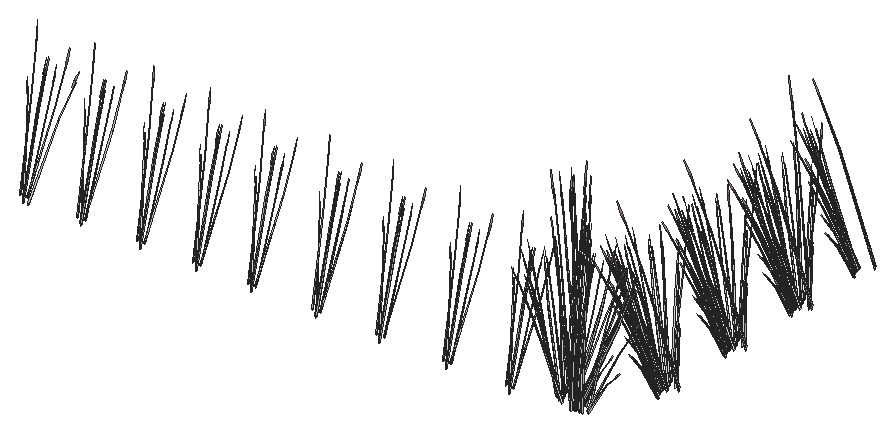
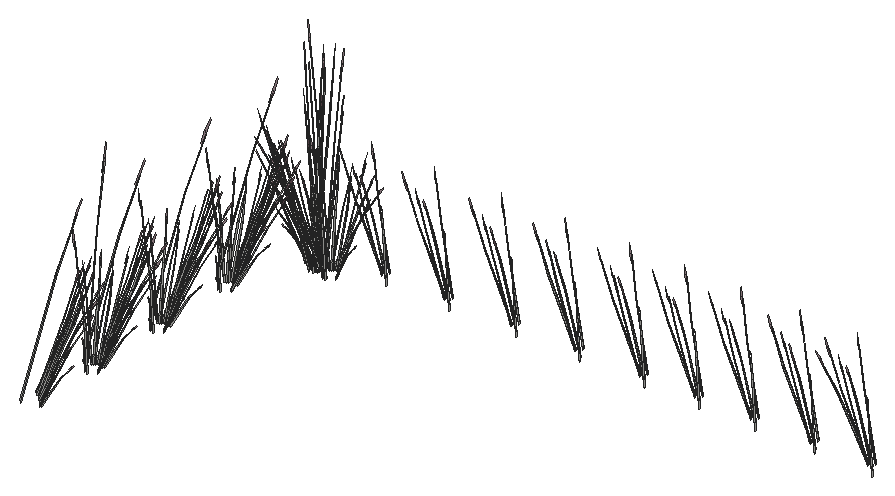
# SketchUp Ruby script. Lengths in inches.
U = 1.inch
M = Sketchup.active_model
def pt(a) = Geom::Point3d.new(a.map { |v| v * U })
def face(e, loops, mat)
  f = e.add_face(loops[0].map { |a| pt(a) })
  loops[1..].each { |l| e.add_face(l.map { |a| pt(a) }).erase! }
  f.material = f.back_material = mat if mat
  f
end
# faces: each face lists its corners as indices into pts; further lists are holes
def faces(e, pts, list, mat = nil) = list.each { |f| face(e, (f[0].is_a?(Array) ? f : [f]).map { |l| l.map { |i| pts[i] } }, mat) }
# xy, xz, yz: faces in a plane at the given z, y or x. An outline is a flat list of corners, or four numbers for a rectangle; further outlines are holes
def ring(l) = l.size == 4 ? [[l[0], l[1]], [l[2], l[1]], [l[2], l[3]], [l[0], l[3]]] : l.each_slice(2).to_a
def flat(e, list, mat, &to3) = list.each { |f| face(e, (f[0].is_a?(Array) ? f : [f]).map { |l| ring(l).map { |u, v| to3.(u, v) } }, mat) }
def xy(e, z, list, mat = nil) = flat(e, list, mat) { |x, y| [x, y, z] }
def xz(e, y, list, mat = nil) = flat(e, list, mat) { |x, z| [x, y, z] }
def yz(e, x, list, mat = nil) = flat(e, list, mat) { |y, z| [x, y, z] }
def lines(e, pts, list) = list.each { |a, b| e.add_line(pt(pts[a]), pt(pts[b])) }
# prism: a flat outline (further loops are holes) pulled along v
def prism(e, loops, v, mat = nil)
  f = face(e, loops, mat); d = Geom::Vector3d.new(v.map { |x| x * U })
  f.pushpull(f.normal.samedirection?(d) ? d.length : -d.length)
end
def box(e, o, s, mat = nil) = prism(e, [[o, [o[0] + s[0], o[1], o[2]], [o[0] + s[0], o[1] + s[1], o[2]], [o[0], o[1] + s[1], o[2]]]], [0, 0, s[2]], mat)
def at(x, y, z, deg = 0) = Geom::Transformation.translation(pt([x, y, z])) * Geom::Transformation.rotation(ORIGIN, Z_AXIS, deg.degrees)
def axes(o, x, y, z) = Geom::Transformation.new([*x, 0, *y, 0, *z, 0, *pt(o).to_a, 1])
def part(name) = M.definitions.add(name)
# library, detail: a bought-in or finely detailed component or shape, given as its bounding box
def library(name, o, s) = part(name).tap { |d| box(d.entities, o, s) }
def detail(e, o, s) = box(e.add_group.entities, o, s)
def put(e, d, t, mat = nil) = e.add_instance(d, t).tap { |i| i.material = mat if mat }
def group(e, t, mat = nil) = e.add_group.tap { |g| g.transformation = t; g.material = mat if mat }.entities
root = M.entities
M.materials.add("LightPink_Translucent").color = [144, 107, 117]
M.materials["LightPink_Translucent"].alpha = 0.75
c1 = part("blade")
p = [[2.15,0.21,22],[0,0.17,0],[0.09,0.45,0],[2.18,0.31,22],[2.29,0.31,22],[0.38,0.45,0],
  [2.48,0.24,33],[2.49,0.24,33],[2.48,0.22,33]]
faces(c1.entities,p,[[0,1,2,3],[4,5,2,3],[6,3,4,7],[8,0,3,6]])
c2 = part("seeds")
p = [[0.3,-0.1,1.38],[-0.01,-0.03,1.59],[-0.01,-0.03,0.03],[0.14,-0.07,-0.07],[0.29,-0.03,3],[0.15,0.01,3.11]]
faces(c2.entities,p,[[0,1,2,3],[1,0,4,5]],"LightPink_Translucent")
c3 = part("blade with seeds")
put(c3.entities,c1,at(0,0,0))
put(c3.entities,c2,axes([2.4,0.25,30.99],[1.5799,-0.05474,1.17369],[-0.12525,1.92788,0.29478],[-0.07173,-0.02425,1.56792]))
put(root,c3,axes([243.23,56.75,257.59],[0.23977,-0.09639,1.43002],[0.59198,0.29065,-0.30754],[-0.1762,0.25149,0.61141]))
put(root,c3,axes([243.82,55.48,260.34],[-0.01977,0.56521,-0.7886],[-0.83252,-0.03796,0.09517],[-0.08786,0.23945,1.11556]))
put(root,c3,axes([243.54,56.28,258.36],[0.01669,-0.31544,1.54345],[0.75083,0.16661,0.21329],[-0.06506,0.33618,0.72882]))
put(root,c3,axes([244.61,55.08,258.875],[-0.0186,-0.23452,1.71376],[0.80601,0.15558,0.13857],[-0.04985,0.33422,0.73262]))
put(root,c3,axes([245.26,56.39,259.53],[-0.22906,0.4699,-0.35414],[-0.66828,-0.13705,0.4572],[0.06128,0.18919,0.87481]))
put(root,c3,axes([245.33,55.97,259.98],[0.36264,0.49684,-0.71045],[-0.74649,0.27689,0.08574],[0.0848,0.24006,1.00501]))
put(root,c3,axes([246.02,54.98,258.875],[-0.17368,-0.19618,1.71376],[0.80256,-0.16516,0.13857],[0.18139,0.30799,0.73262]))
put(root,c3,axes([259.3,56.75,257.59],[0.23977,-0.09639,1.43002],[0.59198,0.29065,-0.30754],[-0.1762,0.25149,0.61141]))
put(root,c3,axes([259.88,55.48,260.34],[-0.01977,0.56521,-0.7886],[-0.83252,-0.03796,0.09517],[-0.08786,0.23945,1.11556]))
put(root,c3,axes([259.61,56.28,258.36],[0.01669,-0.31544,1.54345],[0.75083,0.16661,0.21329],[-0.06506,0.33618,0.72882]))
put(root,c3,axes([260.67,55.08,258.875],[-0.0186,-0.23452,1.71376],[0.80601,0.15558,0.13857],[-0.04985,0.33422,0.73262]))
put(root,c3,axes([261.33,56.39,259.53],[-0.22906,0.4699,-0.35414],[-0.66828,-0.13705,0.4572],[0.06128,0.18919,0.87481]))
put(root,c3,axes([261.39,55.97,259.98],[0.36264,0.49684,-0.71045],[-0.74649,0.27689,0.08574],[0.0848,0.24006,1.00501]))
put(root,c3,axes([276.02,56.75,257.59],[0.23977,-0.09639,1.43002],[0.59198,0.29065,-0.30754],[-0.1762,0.25149,0.61141]))
put(root,c3,axes([276.61,55.48,260.34],[-0.01977,0.56521,-0.7886],[-0.83252,-0.03796,0.09517],[-0.08786,0.23945,1.11556]))
put(root,c3,axes([276.33,56.28,258.36],[0.01669,-0.31544,1.54345],[0.75083,0.16661,0.21329],[-0.06506,0.33618,0.72882]))
put(root,c3,axes([277.4,55.08,258.875],[-0.0186,-0.23452,1.71376],[0.80601,0.15558,0.13857],[-0.04985,0.33422,0.73262]))
put(root,c3,axes([278.05,56.39,259.53],[-0.22906,0.4699,-0.35414],[-0.66828,-0.13705,0.4572],[0.06128,0.18919,0.87481]))
put(root,c3,axes([278.12,55.97,259.98],[0.36264,0.49684,-0.71045],[-0.74649,0.27689,0.08574],[0.0848,0.24006,1.00501]))
put(root,c3,axes([291.75,56.75,257.59],[0.23977,-0.09639,1.43002],[0.59198,0.29065,-0.30754],[-0.1762,0.25149,0.61141]))
put(root,c3,axes([292.34,55.48,260.34],[-0.01977,0.56521,-0.7886],[-0.83252,-0.03796,0.09517],[-0.08786,0.23945,1.11556]))
put(root,c3,axes([292.0625,56.28,258.36],[0.01669,-0.31544,1.54345],[0.75083,0.16661,0.21329],[-0.06506,0.33618,0.72882]))
put(root,c3,axes([293.13,55.08,258.875],[-0.0186,-0.23452,1.71376],[0.80601,0.15558,0.13857],[-0.04985,0.33422,0.73262]))
put(root,c3,axes([293.78,56.39,259.53],[-0.22906,0.4699,-0.35414],[-0.66828,-0.13705,0.4572],[0.06128,0.18919,0.87481]))
put(root,c3,axes([293.85,55.97,259.98],[0.36264,0.49684,-0.71045],[-0.74649,0.27689,0.08574],[0.0848,0.24006,1.00501]))
put(root,c3,axes([307.2,56.75,257.59],[0.23977,-0.09639,1.43002],[0.59198,0.29065,-0.30754],[-0.1762,0.25149,0.61141]))
put(root,c3,axes([307.79,55.48,260.34],[-0.01977,0.56521,-0.7886],[-0.83252,-0.03796,0.09517],[-0.08786,0.23945,1.11556]))
put(root,c3,axes([307.51,56.28,258.36],[0.01669,-0.31544,1.54345],[0.75083,0.16661,0.21329],[-0.06506,0.33618,0.72882]))
put(root,c3,axes([308.58,55.08,258.875],[-0.0186,-0.23452,1.71376],[0.80601,0.15558,0.13857],[-0.04985,0.33422,0.73262]))
put(root,c3,axes([309.23,56.39,259.53],[-0.22906,0.4699,-0.35414],[-0.66828,-0.13705,0.4572],[0.06128,0.18919,0.87481]))
put(root,c3,axes([309.3,55.97,259.98],[0.36264,0.49684,-0.71045],[-0.74649,0.27689,0.08574],[0.0848,0.24006,1.00501]))
put(root,c3,axes([325.31,56.75,257.59],[0.23977,-0.09639,1.43002],[0.59198,0.29065,-0.30754],[-0.1762,0.25149,0.61141]))
put(root,c3,axes([325.9,55.48,260.34],[-0.01977,0.56521,-0.7886],[-0.83252,-0.03796,0.09517],[-0.08786,0.23945,1.11556]))
put(root,c3,axes([325.62,56.28,258.36],[0.01669,-0.31544,1.54345],[0.75083,0.16661,0.21329],[-0.06506,0.33618,0.72882]))
put(root,c3,axes([326.68,55.08,258.875],[-0.0186,-0.23452,1.71376],[0.80601,0.15558,0.13857],[-0.04985,0.33422,0.73262]))
put(root,c3,axes([327.34,56.39,259.53],[-0.22906,0.4699,-0.35414],[-0.66828,-0.13705,0.4572],[0.06128,0.18919,0.87481]))
put(root,c3,axes([327.41,55.97,259.98],[0.36264,0.49684,-0.71045],[-0.74649,0.27689,0.08574],[0.0848,0.24006,1.00501]))
put(root,c3,axes([343.21,56.75,257.59],[0.23977,-0.09639,1.43002],[0.59198,0.29065,-0.30754],[-0.1762,0.25149,0.61141]))
put(root,c3,axes([343.8,55.48,260.34],[-0.01977,0.56521,-0.7886],[-0.83252,-0.03796,0.09517],[-0.08786,0.23945,1.11556]))
put(root,c3,axes([343.52,56.28,258.36],[0.01669,-0.31544,1.54345],[0.75083,0.16661,0.21329],[-0.06506,0.33618,0.72882]))
put(root,c3,axes([344.59,55.08,258.875],[-0.0186,-0.23452,1.71376],[0.80601,0.15558,0.13857],[-0.04985,0.33422,0.73262]))
put(root,c3,axes([345.24,56.39,259.53],[-0.22906,0.4699,-0.35414],[-0.66828,-0.13705,0.4572],[0.06128,0.18919,0.87481]))
put(root,c3,axes([345.3125,55.97,259.98],[0.36264,0.49684,-0.71045],[-0.74649,0.27689,0.08574],[0.0848,0.24006,1.00501]))
put(root,c3,axes([362,56.75,257.59],[0.23977,-0.09639,1.43002],[0.59198,0.29065,-0.30754],[-0.1762,0.25149,0.61141]))
put(root,c3,axes([362.59,55.48,260.34],[-0.01977,0.56521,-0.7886],[-0.83252,-0.03796,0.09517],[-0.08786,0.23945,1.11556]))
put(root,c3,axes([362.31,56.28,258.36],[0.01669,-0.31544,1.54345],[0.75083,0.16661,0.21329],[-0.06506,0.33618,0.72882]))
put(root,c3,axes([363.37,55.08,258.875],[-0.0186,-0.23452,1.71376],[0.80601,0.15558,0.13857],[-0.04985,0.33422,0.73262]))
put(root,c3,axes([364.03,56.39,259.53],[-0.22906,0.4699,-0.35414],[-0.66828,-0.13705,0.4572],[0.06128,0.18919,0.87481]))
put(root,c3,axes([364.1,55.97,259.98],[0.36264,0.49684,-0.71045],[-0.74649,0.27689,0.08574],[0.0848,0.24006,1.00501]))
put(root,c3,axes([379.63,56.75,257.59],[0.23977,-0.09639,1.43002],[0.59198,0.29065,-0.30754],[-0.1762,0.25149,0.61141]))
put(root,c3,axes([380.22,55.48,260.34],[-0.01977,0.56521,-0.7886],[-0.83252,-0.03796,0.09517],[-0.08786,0.23945,1.11556]))
put(root,c3,axes([379.94,56.28,258.36],[0.01669,-0.31544,1.54345],[0.75083,0.16661,0.21329],[-0.06506,0.33618,0.72882]))
put(root,c3,axes([381.01,55.08,258.875],[-0.0186,-0.23452,1.71376],[0.80601,0.15558,0.13857],[-0.04985,0.33422,0.73262]))
put(root,c3,axes([381.66,56.39,259.53],[-0.22906,0.4699,-0.35414],[-0.66828,-0.13705,0.4572],[0.06128,0.18919,0.87481]))
put(root,c3,axes([381.73,55.97,259.98],[0.36264,0.49684,-0.71045],[-0.74649,0.27689,0.08574],[0.0848,0.24006,1.00501]))
put(root,c3,axes([391.02,60,258.875],[0.26363,-0.12925,1.71376],[0.22195,0.59723,0.13857],[-0.41388,0.13498,0.73262]))
put(root,c3,axes([390.2,61.02,257.59],[0.26405,0.05016,1.43002],[0.17019,0.51235,-0.30754],[-0.35868,0.0959,0.61141]))
put(root,c3,axes([392.54,59.375,258.34],[0.21597,-0.08839,1.77064],[0.07448,0.61717,0.13857],[-0.4678,0.08189,0.63284]))
put(root,c3,axes([391.05,59.71,259.68],[-0.20584,0.55581,-0.51099],[-0.70573,-0.19051,-0.3958],[-0.28414,0.05097,0.97773]))
put(root,c3,axes([389.65,62.09,257.77],[0.31665,-0.27694,1.1486],[0.12495,0.43841,0.84392],[-0.22883,0.0785,0.25299]))
put(root,c3,axes([391.99,60.4,258.875],[0.18977,-0.18775,1.71376],[0.47917,0.50677,0.13857],[-0.32866,0.23079,0.73262]))
put(root,c3,axes([390.85,60.89,259.53],[-0.66138,0.08733,-0.35414],[-0.17464,-0.49921,0.4572],[-0.18953,0.13408,0.87481]))
put(root,c3,axes([391.85,60.86,258.875],[0.14147,-0.21002,1.71376],[0.59349,0.43464,0.13857],[-0.26773,0.27089,0.73262]))
put(root,c3,axes([391.39,60.95,259.68],[0.19519,0.55794,-0.51099],[-0.73919,0.0976,-0.3958],[-0.21183,0.14986,0.97773]))
put(root,c3,axes([391.76,62.98,257.59],[0.23977,-0.09639,1.43002],[0.59198,0.29065,-0.30754],[-0.1762,0.25149,0.61141]))
put(root,c3,axes([392.01,62.05,259.53],[-0.5141,0.32171,-0.35414],[-0.48666,-0.36734,0.4572],[-0.07405,0.18664,0.87481]))
put(root,c3,axes([392.35,61.71,260.34],[-0.01977,0.56521,-0.7886],[-0.83252,-0.03796,0.09517],[-0.08786,0.23945,1.11556]))
put(root,c3,axes([392.34,63.3,257.77],[-0.01966,-0.36332,1.1486],[0.49135,0.25914,0.84392],[-0.09663,0.17317,0.25299]))
put(root,c3,axes([393.04,61.77,257.48],[0.7111,0.30552,0.49651],[-0.42504,0.54784,0],[-0.16196,-0.06958,1.57504]))
put(root,c3,axes([392.07,62.5,258.36],[0.01669,-0.31544,1.54345],[0.75083,0.16661,0.21329],[-0.06506,0.33618,0.72882]))
put(root,c3,axes([394.06,60.82,257.62],[-0.14658,0.54532,0.1448],[-0.71613,-0.09466,-0.41347],[-0.13033,-0.05599,1.26744]))
put(root,c3,axes([392.52,61.9,260],[0.54391,0.41056,-0.5672],[-0.57458,0.35956,-0.43934],[-0.08276,0.2086,1.08528]))
put(root,c3,axes([395.72,59.82,257.84],[-0.02076,-0.57531,1.41272],[0.93937,0.14913,0.59816],[-0.22217,0.31481,1.3335]))
put(root,c3,axes([391.93,62.51,257.82],[0.69024,-0.1082,0.06507],[0.15868,0.43593,-0.86304],[-0.04376,0.22067,0.7736]))
put(root,c3,axes([393.14,61.31,258.875],[-0.0186,-0.23452,1.71376],[0.80601,0.15558,0.13857],[-0.04985,0.33422,0.73262]))
put(root,c3,axes([395.74,61.49,257.47],[0.21949,-0.60727,0.17642],[0.8032,0.17185,0.35086],[-0.13875,0.00296,1.60407]))
put(root,c3,axes([395.36,60.6875,257.62],[0.56134,0.36712,0.1448],[-0.46823,0.41419,-0.41347],[-0.13033,0.05599,1.26744]))
put(root,c3,axes([395.35,60.42,257.72],[0.82508,-0.03772,0.44739],[0.07462,0.62614,-0.21531],[-0.14771,0.06346,1.43643]))
put(root,c3,axes([395.96,61.82,257.48],[0.7111,-0.30552,0.49651],[0.42504,0.54784,0],[-0.16196,0.06958,1.57504]))
put(root,c3,axes([393.79,62.62,259.53],[-0.22906,0.4699,-0.35414],[-0.66828,-0.13705,0.4572],[0.06128,0.18919,0.87481]))
put(root,c3,axes([396.99,59.95,257.47],[-0.59697,-0.44509,0.17642],[0.60159,-0.4317,0.35086],[-0.06593,0.0909,1.60407]))
put(root,c3,axes([393.86,62.19,259.98],[0.36264,0.49684,-0.71045],[-0.74649,0.27689,0.08574],[0.0848,0.24006,1.00501]))
put(root,c3,axes([395.55,59.66,257.72],[0.36864,-0.55059,0.44739],[0.76598,0.26498,-0.21531],[0,0.12692,1.43643]))
put(root,c3,axes([394.13,62.29,259.68],[0.7469,0.15318,-0.51099],[-0.25601,0.52518,-0.3958],[0.06849,0.21144,0.97773]))
put(root,c3,axes([395.3,59.52,257.38],[-0.96033,-0.12874,0.49198],[0.19544,-0.7271,0.19306],[0.14034,0.07021,1.70813]))
put(root,c3,axes([395.87,59.78,257.62],[0.70791,-0.1782,0.1448],[0.24791,0.50885,-0.41347],[0,0.11199,1.26744]))
put(root,c3,axes([405.14,146.7,258.875],[0.31515,-0.01384,1.71376],[-0.20907,0.5998,0.13857],[-0.44912,-0.0371,0.73262]))
put(root,c3,axes([397.48,59.96,257.48],[0,-0.61104,0.49651],[0.85008,0,0],[0,0.13917,1.57504]))
put(root,c3,axes([405.42,124.29,258.875],[0.31515,-0.01384,1.71376],[-0.20907,0.5998,0.13857],[-0.44912,-0.0371,0.73262]))
put(root,c3,axes([394.56,61.21,258.875],[-0.17368,-0.19618,1.71376],[0.80256,-0.16516,0.13857],[0.18139,0.30799,0.73262]))
put(root,c3,axes([405.51,77.38,258.875],[0.31515,-0.01384,1.71376],[-0.20907,0.5998,0.13857],[-0.44912,-0.0371,0.73262]))
put(root,c3,axes([405.63,100.9,258.875],[0.31515,-0.01384,1.71376],[-0.20907,0.5998,0.13857],[-0.44912,-0.0371,0.73262]))
put(root,c3,axes([405.55,125.35,258.875],[0.26363,-0.12925,1.71376],[0.22195,0.59723,0.13857],[-0.41388,0.13498,0.73262]))
put(root,c3,axes([405.64,78.43,258.875],[0.26363,-0.12925,1.71376],[0.22195,0.59723,0.13857],[-0.41388,0.13498,0.73262]))
put(root,c3,axes([404.73,126.36,257.59],[0.26405,0.05016,1.43002],[0.17019,0.51235,-0.30754],[-0.35868,0.0959,0.61141]))
put(root,c3,axes([405.76,101.96,258.875],[0.26363,-0.12925,1.71376],[0.22195,0.59723,0.13857],[-0.41388,0.13498,0.73262]))
put(root,c3,axes([404.82,79.45,257.59],[0.26405,0.05016,1.43002],[0.17019,0.51235,-0.30754],[-0.35868,0.0959,0.61141]))
put(root,c3,axes([404.94,102.98,257.59],[0.26405,0.05016,1.43002],[0.17019,0.51235,-0.30754],[-0.35868,0.0959,0.61141]))
put(root,c3,axes([407.0625,124.72,258.34],[0.21597,-0.08839,1.77064],[0.07448,0.61717,0.13857],[-0.4678,0.08189,0.63284]))
put(root,c3,axes([396.77,61.8,257.77],[-0.4278,-0.1757,1.1486],[0.5524,-0.17852,0.84392],[0.14899,0.15122,0.25299]))
put(root,c3,axes([395.24,61.61,257.59],[0.01341,-0.20255,1.43002],[0.64074,-0.22625,-0.30754],[0.1978,0.24243,0.61141]))
put(root,c3,axes([407.15,77.81,258.34],[0.21597,-0.08839,1.77064],[0.07448,0.61717,0.13857],[-0.4678,0.08189,0.63284]))
put(root,c3,axes([407.28,101.34,258.34],[0.21597,-0.08839,1.77064],[0.07448,0.61717,0.13857],[-0.4678,0.08189,0.63284]))
put(root,c3,axes([406.08,146.14,259.98],[-0.75952,-0.01471,-0.71045],[0.05101,-0.61953,0.08574],[-0.32177,-0.06538,1.00501]))
put(root,c3,axes([405.47,146.29,257.59],[0.14835,0.17012,1.43002],[-0.34183,0.46242,-0.30754],[-0.351,-0.11053,0.61141]))
put(root,c3,axes([405.73,145.74,258.875],[0.28223,0.10528,1.71376],[-0.58406,0.44165,0.13857],[-0.36402,-0.19924,0.73262]))
put(root,c3,axes([406.36,123.73,259.98],[-0.75952,-0.01471,-0.71045],[0.05101,-0.61953,0.08574],[-0.32177,-0.06538,1.00501]))
put(root,c3,axes([405.75,123.88,257.59],[0.14835,0.17012,1.43002],[-0.34183,0.46242,-0.30754],[-0.351,-0.11053,0.61141]))
put(root,c3,axes([406.45,76.82,259.98],[-0.75952,-0.01471,-0.71045],[0.05101,-0.61953,0.08574],[-0.32177,-0.06538,1.00501]))
put(root,c3,axes([405.84,76.97,257.59],[0.14835,0.17012,1.43002],[-0.34183,0.46242,-0.30754],[-0.351,-0.11053,0.61141]))
put(root,c3,axes([405.14,124.81,259.53],[-0.63144,-0.17046,-0.35414],[0.18417,-0.49731,0.4572],[-0.25423,0.0456,0.87481]))
put(root,c3,axes([406.58,100.35,259.98],[-0.75952,-0.01471,-0.71045],[0.05101,-0.61953,0.08574],[-0.32177,-0.06538,1.00501]))
put(root,c3,axes([396.83,62.6,257.67],[-0.48723,-0.01916,1.0506],[0.32177,-0.40701,0.58006],[0.19248,0.1446,0.8241]))
put(root,c3,axes([406.01,123.33,258.875],[0.28223,0.10528,1.71376],[-0.58406,0.44165,0.13857],[-0.36402,-0.19924,0.73262]))
put(root,c3,axes([405.96,100.5,257.59],[0.14835,0.17012,1.43002],[-0.34183,0.46242,-0.30754],[-0.351,-0.11053,0.61141]))
put(root,c3,axes([405.23,77.89,259.53],[-0.63144,-0.17046,-0.35414],[0.18417,-0.49731,0.4572],[-0.25423,0.0456,0.87481]))
put(root,c3,axes([406.1,76.42,258.875],[0.28223,0.10528,1.71376],[-0.58406,0.44165,0.13857],[-0.36402,-0.19924,0.73262]))
put(root,c3,axes([405.83,146.27,259.68],[-0.55171,0.40476,-0.51099],[-0.48318,-0.42758,-0.3958],[-0.28031,-0.06159,0.97773]))
put(root,c3,axes([405.36,101.42,259.53],[-0.63144,-0.17046,-0.35414],[0.18417,-0.49731,0.4572],[-0.25423,0.0456,0.87481]))
put(root,c3,axes([406.23,99.94,258.875],[0.28223,0.10528,1.71376],[-0.58406,0.44165,0.13857],[-0.36402,-0.19924,0.73262]))
put(root,c3,axes([405.57,125.06,259.68],[-0.20584,0.55581,-0.51099],[-0.70573,-0.19051,-0.3958],[-0.28414,0.05097,0.97773]))
put(root,c3,axes([405.66,78.15,259.68],[-0.20584,0.55581,-0.51099],[-0.70573,-0.19051,-0.3958],[-0.28414,0.05097,0.97773]))
put(root,c3,axes([406.11,123.86,259.68],[-0.55171,0.40476,-0.51099],[-0.48318,-0.42758,-0.3958],[-0.28031,-0.06159,0.97773]))
put(root,c3,axes([405.79,101.67,259.68],[-0.20584,0.55581,-0.51099],[-0.70573,-0.19051,-0.3958],[-0.28414,0.05097,0.97773]))
put(root,c3,axes([406.2,76.95,259.68],[-0.55171,0.40476,-0.51099],[-0.48318,-0.42758,-0.3958],[-0.28031,-0.06159,0.97773]))
put(root,c3,axes([406.32,100.47,259.68],[-0.55171,0.40476,-0.51099],[-0.48318,-0.42758,-0.3958],[-0.28031,-0.06159,0.97773]))
put(root,c3,axes([404.18,127.4375,257.77],[0.31665,-0.27694,1.1486],[0.12495,0.43841,0.84392],[-0.22883,0.0785,0.25299]))
put(root,c3,axes([395.8,62.04,259.68],[0.74975,-0.14525,-0.51099],[0.13115,0.55007,-0.3958],[0.20138,0.15763,0.97773]))
put(root,c3,axes([405.62,145.89,259.53],[-0.43232,-0.38257,-0.35414],[0.49364,-0.36215,0.4572],[-0.25081,-0.0551,0.87481]))
put(root,c3,axes([404.27,80.52,257.77],[0.31665,-0.27694,1.1486],[0.12495,0.43841,0.84392],[-0.22883,0.0785,0.25299]))
put(root,c3,axes([404.39,104.05,257.77],[0.31665,-0.27694,1.1486],[0.12495,0.43841,0.84392],[-0.22883,0.0785,0.25299]))
put(root,c3,axes([405.9,123.48,259.53],[-0.43232,-0.38257,-0.35414],[0.49364,-0.36215,0.4572],[-0.25081,-0.0551,0.87481]))
put(root,c3,axes([404.58,146.8,257.77],[0.48508,-0.04372,1.1486],[-0.3077,0.38525,0.84392],[-0.23971,-0.05779,0.25299]))
put(root,c3,axes([405.99,76.57,259.53],[-0.43232,-0.38257,-0.35414],[0.49364,-0.36215,0.4572],[-0.25081,-0.0551,0.87481]))
put(root,c3,axes([406.51,125.75,258.875],[0.18977,-0.18775,1.71376],[0.47917,0.50677,0.13857],[-0.32866,0.23079,0.73262]))
put(root,c3,axes([405.37,126.24,259.53],[-0.66138,0.08733,-0.35414],[-0.17464,-0.49921,0.4572],[-0.18953,0.13408,0.87481]))
put(root,c3,axes([406.6,78.84,258.875],[0.18977,-0.18775,1.71376],[0.47917,0.50677,0.13857],[-0.32866,0.23079,0.73262]))
put(root,c3,axes([405.46,79.33,259.53],[-0.66138,0.08733,-0.35414],[-0.17464,-0.49921,0.4572],[-0.18953,0.13408,0.87481]))
put(root,c3,axes([406.12,100.09,259.53],[-0.43232,-0.38257,-0.35414],[0.49364,-0.36215,0.4572],[-0.25081,-0.0551,0.87481]))
put(root,c3,axes([398.5625,61.64,258.93],[-0.14542,-0.51365,-0.03492],[0.68734,-0.11809,-0.15832],[0.14353,0.03256,0.52218]))
put(root,c3,axes([406.73,102.36,258.875],[0.18977,-0.18775,1.71376],[0.47917,0.50677,0.13857],[-0.32866,0.23079,0.73262]))
put(root,c3,axes([404.86,124.4,257.77],[0.48508,-0.04372,1.1486],[-0.3077,0.38525,0.84392],[-0.23971,-0.05779,0.25299]))
put(root,c3,axes([405.59,102.85,259.53],[-0.66138,0.08733,-0.35414],[-0.17464,-0.49921,0.4572],[-0.18953,0.13408,0.87481]))
put(root,c3,axes([404.96,77.48,257.77],[0.48508,-0.04372,1.1486],[-0.3077,0.38525,0.84392],[-0.23971,-0.05779,0.25299]))
put(root,c3,axes([405.08,101.01,257.77],[0.48508,-0.04372,1.1486],[-0.3077,0.38525,0.84392],[-0.23971,-0.05779,0.25299]))
put(root,c3,axes([406.37,126.21,258.875],[0.14147,-0.21002,1.71376],[0.59349,0.43464,0.13857],[-0.26773,0.27089,0.73262]))
put(root,c3,axes([406.46,79.3,258.875],[0.14147,-0.21002,1.71376],[0.59349,0.43464,0.13857],[-0.26773,0.27089,0.73262]))
put(root,c3,axes([395.72,60.6,258.875],[-0.28223,-0.10528,1.71376],[0.58406,-0.44165,0.13857],[0.36402,0.19924,0.73262]))
put(root,c3,axes([406.59,102.82,258.875],[0.14147,-0.21002,1.71376],[0.59349,0.43464,0.13857],[-0.26773,0.27089,0.73262]))
put(root,c3,axes([405.91,126.3,259.68],[0.19519,0.55794,-0.51099],[-0.73919,0.0976,-0.3958],[-0.21183,0.14986,0.97773]))
put(root,c3,axes([406.01,79.39,259.68],[0.19519,0.55794,-0.51099],[-0.73919,0.0976,-0.3958],[-0.21183,0.14986,0.97773]))
put(root,c3,axes([407.4,145.41,259.98],[-0.64788,-0.29534,-0.71045],[0.46044,-0.51755,0.08574],[-0.23473,-0.17635,1.00501]))
put(root,c3,axes([397.27,61.58,259.53],[0.43232,0.38257,-0.35414],[-0.49364,0.36215,0.4572],[0.25081,0.0551,0.87481]))
put(root,c3,axes([407.1,145.43,259.68],[-0.74975,0.14525,-0.51099],[-0.13115,-0.55007,-0.3958],[-0.20138,-0.15763,0.97773]))
put(root,c3,axes([406.13,102.91,259.68],[0.19519,0.55794,-0.51099],[-0.73919,0.0976,-0.3958],[-0.21183,0.14986,0.97773]))
put(root,c3,axes([407.68,123,259.98],[-0.64788,-0.29534,-0.71045],[0.46044,-0.51755,0.08574],[-0.23473,-0.17635,1.00501]))
put(root,c3,axes([407.375,123.02,259.68],[-0.74975,0.14525,-0.51099],[-0.13115,-0.55007,-0.3958],[-0.20138,-0.15763,0.97773]))
put(root,c3,axes([407.77,76.09,259.98],[-0.64788,-0.29534,-0.71045],[0.46044,-0.51755,0.08574],[-0.23473,-0.17635,1.00501]))
put(root,c3,axes([407.47,76.11,259.68],[-0.74975,0.14525,-0.51099],[-0.13115,-0.55007,-0.3958],[-0.20138,-0.15763,0.97773]))
put(root,c3,axes([407.9,99.62,259.98],[-0.64788,-0.29534,-0.71045],[0.46044,-0.51755,0.08574],[-0.23473,-0.17635,1.00501]))
put(root,c3,axes([407.59,99.63,259.68],[-0.74975,0.14525,-0.51099],[-0.13115,-0.55007,-0.3958],[-0.20138,-0.15763,0.97773]))
put(root,c3,axes([399.375,60.35,257.77],[-0.46945,0.10088,1.1486],[0.22097,-0.4169,0.84392],[0.24904,0.02853,0.25299]))
put(root,c3,axes([406.29,128.32,257.59],[0.23977,-0.09639,1.43002],[0.59198,0.29065,-0.30754],[-0.1762,0.25149,0.61141]))
put(root,c3,axes([406.68,144.61,257.59],[-0.04601,0.19989,1.43002],[-0.67263,0.16733,-0.30754],[-0.15723,-0.25836,0.61141]))
put(root,c3,axes([406.38,81.41,257.59],[0.23977,-0.09639,1.43002],[0.59198,0.29065,-0.30754],[-0.1762,0.25149,0.61141]))
put(root,c3,axes([406.9,145.125,258.875],[0.17368,0.19618,1.71376],[-0.80256,0.16516,0.13857],[-0.18139,-0.30799,0.73262]))
put(root,c3,axes([396.82,61.32,259.98],[0.75952,0.01471,-0.71045],[-0.05101,0.61953,0.08574],[0.32177,0.06538,1.00501]))
put(root,c3,axes([406.51,104.9375,257.59],[0.23977,-0.09639,1.43002],[0.59198,0.29065,-0.30754],[-0.1762,0.25149,0.61141]))
put(root,c3,axes([407.18,145.02,259.53],[-0.11735,-0.49217,-0.35414],[0.67083,-0.12996,0.4572],[-0.18018,-0.14104,0.87481]))
put(root,c3,axes([406.95,122.2,257.59],[-0.04601,0.19989,1.43002],[-0.67263,0.16733,-0.30754],[-0.15723,-0.25836,0.61141]))
put(root,c3,axes([407.17,122.72,258.875],[0.17368,0.19618,1.71376],[-0.80256,0.16516,0.13857],[-0.18139,-0.30799,0.73262]))
put(root,c3,axes([407.05,75.29,257.59],[-0.04601,0.19989,1.43002],[-0.67263,0.16733,-0.30754],[-0.15723,-0.25836,0.61141]))
put(root,c3,axes([407.27,75.8,258.875],[0.17368,0.19618,1.71376],[-0.80256,0.16516,0.13857],[-0.18139,-0.30799,0.73262]))
put(root,c3,axes([407.17,98.8125,257.59],[-0.04601,0.19989,1.43002],[-0.67263,0.16733,-0.30754],[-0.15723,-0.25836,0.61141]))
put(root,c3,axes([407.45,122.61,259.53],[-0.11735,-0.49217,-0.35414],[0.67083,-0.12996,0.4572],[-0.18018,-0.14104,0.87481]))
put(root,c3,axes([407.39,99.33,258.875],[0.17368,0.19618,1.71376],[-0.80256,0.16516,0.13857],[-0.18139,-0.30799,0.73262]))
put(root,c3,axes([407.55,75.7,259.53],[-0.11735,-0.49217,-0.35414],[0.67083,-0.12996,0.4572],[-0.18018,-0.14104,0.87481]))
put(root,c3,axes([406.53,127.4,259.53],[-0.5141,0.32171,-0.35414],[-0.48666,-0.36734,0.4572],[-0.07405,0.18664,0.87481]))
put(root,c3,axes([407.67,99.23,259.53],[-0.11735,-0.49217,-0.35414],[0.67083,-0.12996,0.4572],[-0.18018,-0.14104,0.87481]))
put(root,c3,axes([406.625,80.48,259.53],[-0.5141,0.32171,-0.35414],[-0.48666,-0.36734,0.4572],[-0.07405,0.18664,0.87481]))
put(root,c3,axes([408.95,148.75,258.33],[0.65659,0.2464,1.51261],[-0.64324,0.53082,0.59816],[-0.28812,-0.31461,1.26806]))
put(root,c3,axes([406.75,104.01,259.53],[-0.5141,0.32171,-0.35414],[-0.48666,-0.36734,0.4572],[-0.07405,0.18664,0.87481]))
put(root,c3,axes([406.44,144.29,257.77],[0.39634,0.21267,1.1486],[-0.57721,0.12784,0.84392],[-0.1235,-0.16344,0.25299]))
put(root,c3,axes([409.23,126.34,258.33],[0.65659,0.2464,1.51261],[-0.64324,0.53082,0.59816],[-0.28812,-0.31461,1.26806]))
put(root,c3,axes([409.32,79.43,258.33],[0.65659,0.2464,1.51261],[-0.64324,0.53082,0.59816],[-0.28812,-0.31461,1.26806]))
put(root,c3,axes([406.72,121.875,257.77],[0.39634,0.21267,1.1486],[-0.57721,0.12784,0.84392],[-0.1235,-0.16344,0.25299]))
put(root,c3,axes([398.5,61.02,257.59],[-0.18299,-0.15028,1.43002],[0.23809,-0.49714,-0.30754],[0.37023,0.06735,0.61141]))
put(root,c3,axes([406.82,74.96,257.77],[0.39634,0.21267,1.1486],[-0.57721,0.12784,0.84392],[-0.1235,-0.16344,0.25299]))
put(root,c3,axes([409.45,102.96,258.33],[0.65659,0.2464,1.51261],[-0.64324,0.53082,0.59816],[-0.28812,-0.31461,1.26806]))
put(root,c3,axes([406.875,127.06,260.34],[-0.01977,0.56521,-0.7886],[-0.83252,-0.03796,0.09517],[-0.08786,0.23945,1.11556]))
put(root,c3,axes([406.94,98.49,257.77],[0.39634,0.21267,1.1486],[-0.57721,0.12784,0.84392],[-0.1235,-0.16344,0.25299]))
put(root,c3,axes([406.97,80.14,260.34],[-0.01977,0.56521,-0.7886],[-0.83252,-0.03796,0.09517],[-0.08786,0.23945,1.11556]))
put(root,c3,axes([406.86,128.65,257.77],[-0.01966,-0.36332,1.1486],[0.49135,0.25914,0.84392],[-0.09663,0.17317,0.25299]))
put(root,c3,axes([406.95,81.73,257.77],[-0.01966,-0.36332,1.1486],[0.49135,0.25914,0.84392],[-0.09663,0.17317,0.25299]))
put(root,c3,axes([407.09,103.67,260.34],[-0.01977,0.56521,-0.7886],[-0.83252,-0.03796,0.09517],[-0.08786,0.23945,1.11556]))
put(root,c3,axes([407.08,105.26,257.77],[-0.01966,-0.36332,1.1486],[0.49135,0.25914,0.84392],[-0.09663,0.17317,0.25299]))
put(root,c3,axes([407.5625,127.12,257.48],[0.7111,0.30552,0.49651],[-0.42504,0.54784,0],[-0.16196,-0.06958,1.57504]))
